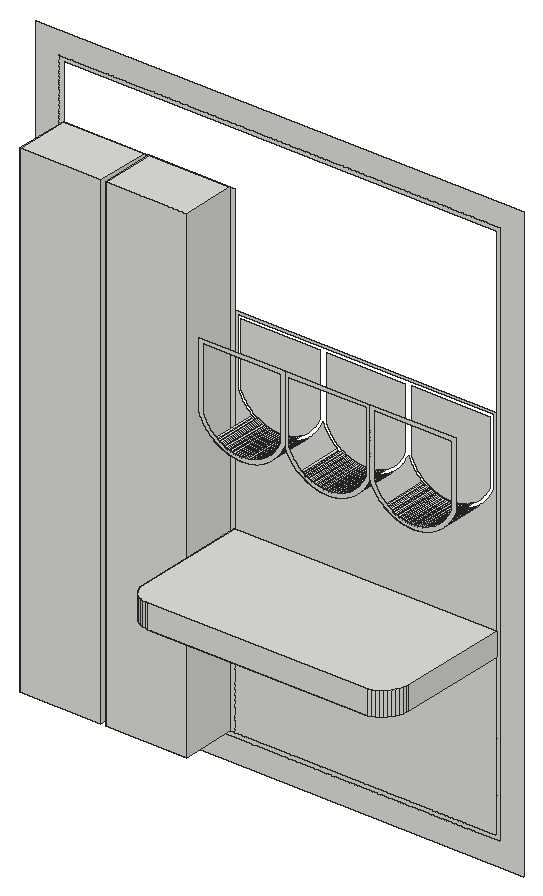
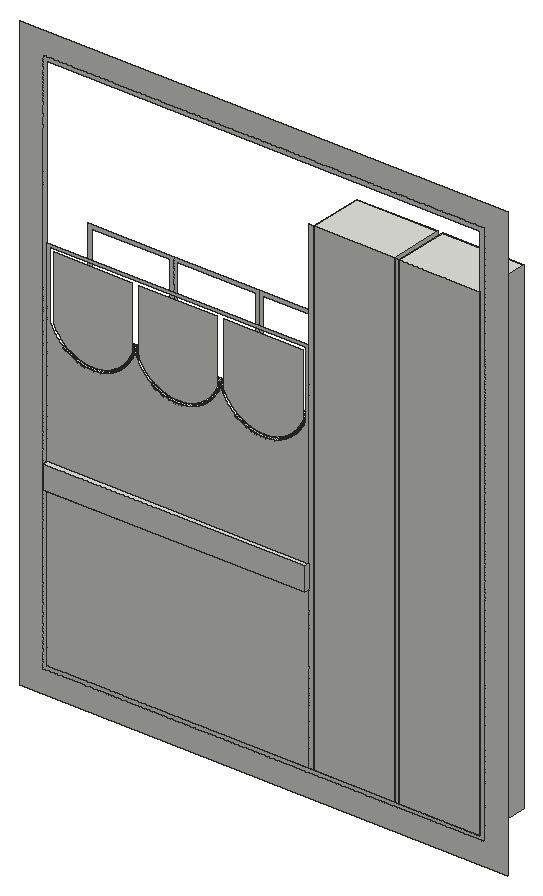
# SketchUp Ruby script. Lengths in inches.
U = 1.inch
M = Sketchup.active_model
def pt(a) = Geom::Point3d.new(a.map { |v| v * U })
def face(e, loops, mat)
  f = e.add_face(loops[0].map { |a| pt(a) })
  loops[1..].each { |l| e.add_face(l.map { |a| pt(a) }).erase! }
  f.material = f.back_material = mat if mat
  f
end
# faces: each face lists its corners as indices into pts; further lists are holes
def faces(e, pts, list, mat = nil) = list.each { |f| face(e, (f[0].is_a?(Array) ? f : [f]).map { |l| l.map { |i| pts[i] } }, mat) }
# xy, xz, yz: faces in a plane at the given z, y or x. An outline is a flat list of corners, or four numbers for a rectangle; further outlines are holes
def ring(l) = l.size == 4 ? [[l[0], l[1]], [l[2], l[1]], [l[2], l[3]], [l[0], l[3]]] : l.each_slice(2).to_a
def flat(e, list, mat, &to3) = list.each { |f| face(e, (f[0].is_a?(Array) ? f : [f]).map { |l| ring(l).map { |u, v| to3.(u, v) } }, mat) }
def xy(e, z, list, mat = nil) = flat(e, list, mat) { |x, y| [x, y, z] }
def xz(e, y, list, mat = nil) = flat(e, list, mat) { |x, z| [x, y, z] }
def yz(e, x, list, mat = nil) = flat(e, list, mat) { |y, z| [x, y, z] }
def lines(e, pts, list) = list.each { |a, b| e.add_line(pt(pts[a]), pt(pts[b])) }
# prism: a flat outline (further loops are holes) pulled along v
def prism(e, loops, v, mat = nil)
  f = face(e, loops, mat); d = Geom::Vector3d.new(v.map { |x| x * U })
  f.pushpull(f.normal.samedirection?(d) ? d.length : -d.length)
end
def box(e, o, s, mat = nil) = prism(e, [[o, [o[0] + s[0], o[1], o[2]], [o[0] + s[0], o[1] + s[1], o[2]], [o[0], o[1] + s[1], o[2]]]], [0, 0, s[2]], mat)
def at(x, y, z, deg = 0) = Geom::Transformation.translation(pt([x, y, z])) * Geom::Transformation.rotation(ORIGIN, Z_AXIS, deg.degrees)
def axes(o, x, y, z) = Geom::Transformation.new([*x, 0, *y, 0, *z, 0, *pt(o).to_a, 1])
def part(name) = M.definitions.add(name)
# library, detail: a bought-in or finely detailed component or shape, given as its bounding box
def library(name, o, s) = part(name).tap { |d| box(d.entities, o, s) }
def detail(e, o, s) = box(e.add_group.entities, o, s)
def put(e, d, t, mat = nil) = e.add_instance(d, t).tap { |i| i.material = mat if mat }
def group(e, t, mat = nil) = e.add_group.tap { |g| g.transformation = t; g.material = mat if mat }.entities
root = M.entities
xy(root,62.04,[[91.5625,19.34,91.81,30],[91.81,19.34,92.06,30],[92.06,19.34,92.3,30]])
xy(root,62.1,[[72.875,19.34,73.125,30]])
xy(root,62.12,[[53.94,19.34,54.19,30]])
xy(root,62.84,[[91.59,19.34,91.82,30],[91.82,19.34,92.05,30],[92.05,19.34,92.28,30]])
xy(root,62.9,[[72.89,19.34,73.11,30]])
xy(root,62.92,[[53.73,19.34,53.95,30],[53.95,19.34,54.18,30],[54.18,19.34,54.41,30]])
xz(root,19.34,[[[91.5625,62.04,92.3,62.04,92.55,62.06,92.8,62.07,93.05,62.1,93.29,62.13,93.54,62.17,93.78,62.21,94.26,62.31,94.5,62.37,94.74,62.4375,94.98,62.51,95.22,62.59,95.45,62.67,95.91,62.85,96.13,62.95,96.36,63.06,96.58,63.17,96.8,63.29,97.01,63.41,97.23,63.53,97.4375,63.67,97.64,63.8,97.84,63.95,98.04,64.09,98.24,64.25,98.43,64.4,98.62,64.5625,98.8,64.73,99.16,65.07,99.33,65.25,99.49,65.4375,99.66,65.625,99.8125,65.81,99.97,66.01,100.11,66.21,100.26,66.41,100.4,66.62,100.53,66.82,100.66,67.04,100.78,67.25,100.9,67.47,101.01,67.69,101.11,67.91,101.15,68,101.21,68.14,101.31,68.37,101.4,68.6,101.4,83.4,82.47,83.4,82.47,68.6,82.65,68.14,82.71,68,82.75,67.91,82.97,67.47,83.09,67.25,83.21,67.04,83.34,66.82,83.47,66.62,83.61,66.41,83.75,66.21,84.05,65.81,84.21,65.625,84.37,65.4375,84.54,65.25,84.71,65.07,84.89,64.9,85.06,64.73,85.25,64.5625,85.4375,64.4,85.63,64.25,85.82,64.09,86.02,63.95,86.22,63.8,86.43,63.67,86.64,63.53,86.85,63.41,87.29,63.17,87.73,62.95,87.96,62.85,88.1875,62.76,88.42,62.67,88.65,62.59,88.89,62.51,89.125,62.4375,89.36,62.37,89.6,62.31,89.84,62.26,90.09,62.21,90.33,62.17,90.58,62.13,90.82,62.1,91.07,62.07,91.31,62.06],[91.59,62.84,91.36,62.86,91.14,62.87,90.91,62.89,90.68,62.92,90.46,62.96,90.23,62.99,89.57,63.14,89.35,63.2,88.91,63.34,88.7,63.42,88.48,63.5,88.27,63.59,88.0625,63.68,87.86,63.78,87.65,63.88,87.25,64.1,86.68,64.46,86.49,64.59,86.31,64.73,86.125,64.87,85.95,65.01,85.78,65.16,85.61,65.32,85.44,65.47,85.28,65.63,84.97,65.97,84.82,66.14,84.4,66.68,84.27,66.86,84.14,67.05,84.02,67.25,83.9,67.44,83.68,67.84,83.58,68.04,83.48,68.25,83.45,68.33,83.39,68.46,83.3,68.67,83.27,68.75,83.27,82.6,100.6,82.6,100.6,68.75,100.57,68.67,100.48,68.46,100.42,68.33,100.39,68.25,100.29,68.04,100.1875,67.84,100.08,67.64,99.97,67.44,99.85,67.25,99.73,67.05,99.6,66.86,99.47,66.68,99.05,66.14,98.9,65.97,98.74,65.8,98.59,65.63,98.42,65.47,98.26,65.32,98.09,65.16,97.92,65.01,97.56,64.73,97.375,64.59,97.19,64.46,96.81,64.22,96.61,64.1,96.21,63.88,96.01,63.78,95.8,63.68,95.38,63.5,94.96,63.34,94.52,63.2,94.3,63.14,93.86,63.04,93.63,62.99,93.41,62.96,93.18,62.92,92.96,62.89,92.73,62.87,92.5,62.86,92.28,62.84]],[[72.875,62.1,73.125,62.1,73.37,62.11,73.62,62.12,73.86,62.14,74.11,62.16,74.35,62.1875,74.6,62.23,75.08,62.31,75.32,62.37,75.5625,62.43,75.8,62.49,76.04,62.5625,76.27,62.64,76.5,62.72,76.73,62.8125,76.96,62.9,77.1875,63,77.41,63.11,77.85,63.33,78.0625,63.45,78.28,63.58,78.49,63.71,79.09,64.13,79.29,64.28,79.48,64.4375,79.67,64.6,79.85,64.76,80.21,65.1,80.55,65.46,80.87,65.84,81.02,66.03,81.17,66.23,81.3125,66.43,81.45,66.63,81.84,67.26,81.96,67.48,82.18,67.92,82.21,68,82.28,68.14,82.47,68.6,82.47,83.4,63.53,83.4,63.53,68.6,63.72,68.14,63.79,68,63.82,67.92,64.04,67.48,64.16,67.26,64.55,66.63,64.6875,66.43,64.83,66.23,64.98,66.03,65.13,65.84,65.45,65.46,65.79,65.1,66.15,64.76,66.33,64.6,66.52,64.4375,66.71,64.28,66.91,64.13,67.51,63.71,67.72,63.58,67.9375,63.45,68.15,63.33,68.59,63.11,68.8125,63,69.04,62.9,69.27,62.8125,69.5,62.72,69.73,62.64,69.96,62.5625,70.2,62.49,70.4375,62.43,70.68,62.37,70.92,62.31,71.4,62.23,71.65,62.1875,71.89,62.16,72.14,62.14,72.38,62.12,72.63,62.11],[72.89,62.9,72.43,62.92,72.21,62.93,71.98,62.95,71.75,62.98,71.53,63.02,71.31,63.05,71.08,63.1,70.64,63.2,70.42,63.26,70.2,63.33,69.99,63.4,69.77,63.47,69.5625,63.55,69.35,63.64,69.14,63.73,68.9375,63.83,68.73,63.93,68.53,64.04,68.34,64.15,68.14,64.26,67.95,64.38,67.57,64.64,67.39,64.77,67.03,65.05,66.86,65.2,66.6875,65.35,66.52,65.51,66.2,65.83,65.75,66.34,65.61,66.52,65.48,66.7,65.34,66.89,65.22,67.07,65.09,67.27,64.97,67.46,64.86,67.66,64.75,67.85,64.65,68.06,64.55,68.26,64.52,68.33,64.45,68.47,64.33,68.75,64.33,82.6,81.67,82.6,81.67,68.75,81.55,68.47,81.48,68.33,81.45,68.26,81.35,68.06,81.25,67.85,81.14,67.66,81.03,67.46,80.91,67.27,80.78,67.07,80.66,66.89,80.52,66.7,80.39,66.52,80.25,66.34,79.8,65.83,79.48,65.51,79.3125,65.35,79.14,65.2,78.97,65.05,78.61,64.77,78.43,64.64,78.05,64.38,77.86,64.26,77.66,64.15,77.47,64.04,77.27,63.93,77.0625,63.83,76.86,63.73,76.65,63.64,76.4375,63.55,76.23,63.47,76.01,63.4,75.8,63.33,75.58,63.26,75.36,63.2,74.92,63.1,74.69,63.05,74.47,63.02,74.25,62.98,74.02,62.95,73.79,62.93,73.57,62.92,73.11,62.9]],[[53.94,62.12,54.19,62.12,54.4375,62.125,54.68,62.14,54.93,62.15,55.17,62.18,55.42,62.21,55.66,62.24,55.9,62.29,56.15,62.33,56.39,62.39,56.86,62.51,57.1,62.58,57.33,62.66,57.57,62.74,57.8,62.83,58.02,62.92,58.25,63.02,58.69,63.23,58.91,63.35,59.34,63.59,59.55,63.72,60.15,64.14,60.35,64.29,60.73,64.61,60.91,64.77,61.27,65.11,61.61,65.47,61.77,65.66,61.93,65.84,62.08,66.04,62.23,66.23,62.375,66.43,62.51,66.64,62.65,66.84,62.78,67.05,62.9,67.27,63.02,67.48,63.28,68,63.34,68.15,63.44,68.37,63.53,68.6,63.53,83.4,44.6,83.4,44.6,68.6,44.69,68.37,44.79,68.15,44.86,68,44.89,67.92,45.11,67.48,45.23,67.27,45.36,67.05,45.49,66.84,45.62,66.64,45.76,66.43,45.9,66.23,46.05,66.04,46.21,65.84,46.36,65.66,46.53,65.47,46.69,65.29,47.04,64.94,47.22,64.77,47.4,64.61,47.78,64.29,47.98,64.14,48.38,63.86,48.59,63.72,48.8,63.59,49.22,63.35,49.44,63.23,49.88,63.02,50.11,62.92,50.57,62.74,51.03,62.58,51.27,62.51,51.99,62.33,52.23,62.29,52.47,62.24,52.72,62.21,52.96,62.18,53.21,62.15,53.45,62.14,53.7,62.125],[53.73,62.92,53.5,62.93,53.27,62.95,53.05,62.97,52.82,63,52.6,63.03,52.375,63.07,52.15,63.12,51.93,63.16,51.27,63.34,51.06,63.41,50.84,63.49,50.63,63.57,50.21,63.75,50.01,63.84,49.81,63.94,49.6,64.05,49.41,64.16,49.21,64.28,48.83,64.52,48.64,64.65,48.46,64.78,48.28,64.92,48.1,65.07,47.93,65.21,47.76,65.36,47.59,65.52,47.27,65.84,46.97,66.18,46.83,66.35,46.68,66.53,46.55,66.71,46.41,66.89,46.29,67.08,46.16,67.27,46.04,67.46,45.71,68.06,45.61,68.26,45.4,68.75,45.4,82.6,62.73,82.6,62.73,68.75,62.52,68.26,62.42,68.06,62.3125,67.86,62.2,67.66,62.09,67.46,61.85,67.08,61.72,66.89,61.59,66.71,61.31,66.35,60.86,65.84,60.54,65.52,60.375,65.36,60.2,65.21,60.03,65.07,59.85,64.92,59.67,64.78,59.49,64.65,59.3,64.52,58.73,64.16,58.33,63.94,58.125,63.84,57.92,63.75,57.5,63.57,57.08,63.41,56.86,63.34,56.2,63.16,55.98,63.12,55.76,63.07,55.54,63.03,55.3125,63,55.09,62.97,54.63,62.93,54.41,62.92]]])
xz(root,30,[[[0,-6,108,126],[5,-1,103,121]],[[5,-1,103,121],[6,0,102,120]],[24,0,25,108],[43,0,44,108],[44,0,102,35.4],
  [[44,40.6,102,84],[91.5625,62.04,91.31,62.06,91.07,62.07,90.82,62.1,90.58,62.13,90.33,62.17,90.09,62.21,89.84,62.26,89.6,62.31,89.36,62.37,89.125,62.4375,88.89,62.51,88.65,62.59,88.42,62.67,88.1875,62.76,87.96,62.85,87.73,62.95,87.29,63.17,86.85,63.41,86.64,63.53,86.43,63.67,86.22,63.8,86.02,63.95,85.82,64.09,85.63,64.25,85.4375,64.4,85.25,64.5625,85.06,64.73,84.89,64.9,84.71,65.07,84.54,65.25,84.37,65.4375,84.21,65.625,84.05,65.81,83.75,66.21,83.61,66.41,83.47,66.62,83.34,66.82,83.21,67.04,83.09,67.25,82.97,67.47,82.75,67.91,82.71,68,82.65,68.14,82.47,68.6,82.28,68.14,82.21,68,82.18,67.92,81.96,67.48,81.84,67.26,81.45,66.63,81.3125,66.43,81.17,66.23,81.02,66.03,80.87,65.84,80.55,65.46,80.21,65.1,79.85,64.76,79.67,64.6,79.48,64.4375,79.29,64.28,79.09,64.13,78.49,63.71,78.28,63.58,78.0625,63.45,77.85,63.33,77.41,63.11,77.1875,63,76.96,62.9,76.73,62.8125,76.5,62.72,76.27,62.64,76.04,62.5625,75.8,62.49,75.5625,62.43,75.32,62.37,75.08,62.31,74.6,62.23,74.35,62.1875,74.11,62.16,73.86,62.14,73.62,62.12,73.37,62.11,73.125,62.1,72.875,62.1,72.63,62.11,72.38,62.12,72.14,62.14,71.89,62.16,71.65,62.1875,71.4,62.23,70.92,62.31,70.68,62.37,70.4375,62.43,70.2,62.49,69.96,62.5625,69.73,62.64,69.5,62.72,69.27,62.8125,69.04,62.9,68.8125,63,68.59,63.11,68.15,63.33,67.9375,63.45,67.72,63.58,67.51,63.71,66.91,64.13,66.71,64.28,66.52,64.4375,66.33,64.6,66.15,64.76,65.79,65.1,65.45,65.46,65.13,65.84,64.98,66.03,64.83,66.23,64.6875,66.43,64.55,66.63,64.16,67.26,64.04,67.48,63.82,67.92,63.79,68,63.72,68.14,63.53,68.6,63.44,68.37,63.34,68.15,63.28,68,63.02,67.48,62.9,67.27,62.78,67.05,62.65,66.84,62.51,66.64,62.375,66.43,62.23,66.23,62.08,66.04,61.93,65.84,61.77,65.66,61.61,65.47,61.27,65.11,60.91,64.77,60.73,64.61,60.35,64.29,60.15,64.14,59.55,63.72,59.34,63.59,58.91,63.35,58.69,63.23,58.25,63.02,58.02,62.92,57.8,62.83,57.57,62.74,57.33,62.66,57.1,62.58,56.86,62.51,56.39,62.39,56.15,62.33,55.9,62.29,55.66,62.24,55.42,62.21,55.17,62.18,54.93,62.15,54.68,62.14,54.4375,62.125,54.19,62.12,53.94,62.12,53.7,62.125,53.45,62.14,53.21,62.15,52.96,62.18,52.72,62.21,52.47,62.24,52.23,62.29,51.99,62.33,51.27,62.51,51.03,62.58,50.57,62.74,50.11,62.92,49.88,63.02,49.44,63.23,49.22,63.35,48.8,63.59,48.59,63.72,48.38,63.86,47.98,64.14,47.78,64.29,47.4,64.61,47.22,64.77,47.04,64.94,46.69,65.29,46.53,65.47,46.36,65.66,46.21,65.84,46.05,66.04,45.9,66.23,45.76,66.43,45.62,66.64,45.49,66.84,45.36,67.05,45.23,67.27,45.11,67.48,44.89,67.92,44.86,68,44.79,68.15,44.69,68.37,44.6,68.6,44.6,83.4,101.4,83.4,101.4,68.6,101.31,68.37,101.21,68.14,101.15,68,101.11,67.91,101.01,67.69,100.9,67.47,100.78,67.25,100.66,67.04,100.53,66.82,100.4,66.62,100.26,66.41,100.11,66.21,99.97,66.01,99.8125,65.81,99.66,65.625,99.49,65.4375,99.33,65.25,99.16,65.07,98.8,64.73,98.62,64.5625,98.43,64.4,98.24,64.25,98.04,64.09,97.84,63.95,97.64,63.8,97.4375,63.67,97.23,63.53,97.01,63.41,96.8,63.29,96.58,63.17,96.36,63.06,96.13,62.95,95.91,62.85,95.45,62.67,95.22,62.59,94.98,62.51,94.74,62.4375,94.5,62.37,94.26,62.31,93.78,62.21,93.54,62.17,93.29,62.13,93.05,62.1,92.8,62.07,92.55,62.06,92.3,62.04]],[91.59,62.84,92.28,62.84,92.5,62.86,92.73,62.87,92.96,62.89,93.18,62.92,93.41,62.96,93.63,62.99,93.86,63.04,94.3,63.14,94.52,63.2,94.96,63.34,95.38,63.5,95.8,63.68,96.01,63.78,96.21,63.88,96.61,64.1,96.81,64.22,97.19,64.46,97.375,64.59,97.56,64.73,97.92,65.01,98.09,65.16,98.26,65.32,98.42,65.47,98.59,65.63,98.74,65.8,98.9,65.97,99.05,66.14,99.47,66.68,99.6,66.86,99.73,67.05,99.85,67.25,99.97,67.44,100.08,67.64,100.1875,67.84,100.29,68.04,100.39,68.25,100.42,68.33,100.48,68.46,100.57,68.67,100.6,68.75,100.6,82.6,83.27,82.6,83.27,68.75,83.3,68.67,83.39,68.46,83.45,68.33,83.48,68.25,83.58,68.04,83.68,67.84,83.9,67.44,84.02,67.25,84.14,67.05,84.27,66.86,84.4,66.68,84.82,66.14,84.97,65.97,85.28,65.63,85.44,65.47,85.61,65.32,85.78,65.16,85.95,65.01,86.125,64.87,86.31,64.73,86.49,64.59,86.68,64.46,87.25,64.1,87.65,63.88,87.86,63.78,88.0625,63.68,88.27,63.59,88.48,63.5,88.7,63.42,88.91,63.34,89.35,63.2,89.57,63.14,90.23,62.99,90.46,62.96,90.68,62.92,90.91,62.89,91.14,62.87,91.36,62.86],[72.89,62.9,73.11,62.9,73.57,62.92,73.79,62.93,74.02,62.95,74.25,62.98,74.47,63.02,74.69,63.05,74.92,63.1,75.36,63.2,75.58,63.26,75.8,63.33,76.01,63.4,76.23,63.47,76.4375,63.55,76.65,63.64,76.86,63.73,77.0625,63.83,77.27,63.93,77.47,64.04,77.66,64.15,77.86,64.26,78.05,64.38,78.43,64.64,78.61,64.77,78.97,65.05,79.14,65.2,79.3125,65.35,79.48,65.51,79.8,65.83,80.25,66.34,80.39,66.52,80.52,66.7,80.66,66.89,80.78,67.07,80.91,67.27,81.03,67.46,81.14,67.66,81.25,67.85,81.35,68.06,81.45,68.26,81.48,68.33,81.55,68.47,81.67,68.75,81.67,82.6,64.33,82.6,64.33,68.75,64.45,68.47,64.52,68.33,64.55,68.26,64.65,68.06,64.75,67.85,64.86,67.66,64.97,67.46,65.09,67.27,65.22,67.07,65.34,66.89,65.48,66.7,65.61,66.52,65.75,66.34,66.2,65.83,66.52,65.51,66.6875,65.35,66.86,65.2,67.03,65.05,67.39,64.77,67.57,64.64,67.95,64.38,68.14,64.26,68.34,64.15,68.53,64.04,68.73,63.93,68.9375,63.83,69.14,63.73,69.35,63.64,69.5625,63.55,69.77,63.47,69.99,63.4,70.2,63.33,70.42,63.26,70.64,63.2,71.08,63.1,71.31,63.05,71.53,63.02,71.75,62.98,71.98,62.95,72.21,62.93,72.43,62.92],[53.73,62.92,54.41,62.92,54.63,62.93,55.09,62.97,55.3125,63,55.54,63.03,55.76,63.07,55.98,63.12,56.2,63.16,56.86,63.34,57.08,63.41,57.5,63.57,57.92,63.75,58.125,63.84,58.33,63.94,58.73,64.16,59.3,64.52,59.49,64.65,59.67,64.78,59.85,64.92,60.03,65.07,60.2,65.21,60.375,65.36,60.54,65.52,60.86,65.84,61.31,66.35,61.59,66.71,61.72,66.89,61.85,67.08,62.09,67.46,62.2,67.66,62.3125,67.86,62.42,68.06,62.52,68.26,62.73,68.75,62.73,82.6,45.4,82.6,45.4,68.75,45.61,68.26,45.71,68.06,46.04,67.46,46.16,67.27,46.29,67.08,46.41,66.89,46.55,66.71,46.68,66.53,46.83,66.35,46.97,66.18,47.27,65.84,47.59,65.52,47.76,65.36,47.93,65.21,48.1,65.07,48.28,64.92,48.46,64.78,48.64,64.65,48.83,64.52,49.21,64.28,49.41,64.16,49.6,64.05,49.81,63.94,50.01,63.84,50.21,63.75,50.63,63.57,50.84,63.49,51.06,63.41,51.27,63.34,51.93,63.16,52.15,63.12,52.375,63.07,52.6,63.03,52.82,63,53.05,62.97,53.27,62.95,53.5,62.93]])
p = [[91.31,30,62.06],[91.5625,30,62.04],[91.5625,19.34,62.04],[91.31,19.34,62.06],[92.3,30,62.04],[92.55,30,62.06],
  [92.55,19.34,62.06],[92.3,19.34,62.04],[53.21,30,62.15],[53.45,30,62.14],[53.45,19.34,62.14],[53.21,19.34,62.15],
  [53.7,30,62.125],[53.7,19.34,62.125],[53.94,30,62.12],[53.94,19.34,62.12],[54.19,30,62.12],[54.4375,30,62.125],
  [54.4375,19.34,62.125],[54.19,19.34,62.12],[54.68,30,62.14],[54.68,19.34,62.14],[54.93,30,62.15],[54.93,19.34,62.15],
  [71.89,30,62.16],[72.14,30,62.14],[72.14,19.34,62.14],[71.89,19.34,62.16],[72.38,30,62.12],[72.38,19.34,62.12],
  [72.63,30,62.11],[72.63,19.34,62.11],[72.875,30,62.1],[72.875,19.34,62.1],[73.125,30,62.1],[73.37,30,62.11],
  [73.37,19.34,62.11],[73.125,19.34,62.1],[73.62,30,62.12],[73.62,19.34,62.12],[73.86,30,62.14],[73.86,19.34,62.14],
  [74.11,30,62.16],[74.11,19.34,62.16],[90.33,30,62.17],[90.58,30,62.13],[90.58,19.34,62.13],[90.33,19.34,62.17],
  [90.82,30,62.1],[90.82,19.34,62.1],[91.07,30,62.07],[91.07,19.34,62.07],[92.8,30,62.07],[92.8,19.34,62.07],
  [93.05,30,62.1],[93.05,19.34,62.1],[93.29,30,62.13],[93.29,19.34,62.13],[93.54,30,62.17],[93.54,19.34,62.17],
  [52.23,30,62.29],[52.47,30,62.24],[52.47,19.34,62.24],[52.23,19.34,62.29],[52.72,30,62.21],[52.72,19.34,62.21],
  [52.96,30,62.18],[52.96,19.34,62.18],[55.17,30,62.18],[55.17,19.34,62.18],[55.42,30,62.21],[55.42,19.34,62.21],
  [55.66,30,62.24],[55.66,19.34,62.24],[55.9,30,62.29],[55.9,19.34,62.29],[71.16,30,62.27],[71.4,30,62.23],
  [71.4,19.34,62.23],[71.16,19.34,62.27],[71.65,30,62.1875],[71.65,19.34,62.1875],[74.35,30,62.1875],[74.35,19.34,62.1875],
  [74.6,30,62.23],[74.6,19.34,62.23],[74.84,30,62.27],[74.84,19.34,62.27],[89.84,30,62.26],[90.09,30,62.21],
  [90.09,19.34,62.21],[89.84,19.34,62.26],[93.78,30,62.21],[93.78,19.34,62.21],[94.02,30,62.26],[94.02,19.34,62.26],
  [51.75,30,62.39],[51.99,30,62.33],[51.99,19.34,62.33],[51.75,19.34,62.39],[56.15,30,62.33],[56.15,19.34,62.33],
  [56.39,30,62.39],[56.39,19.34,62.39],[70.68,30,62.37],[70.92,30,62.31],[70.92,19.34,62.31],[70.68,19.34,62.37],
  [75.08,30,62.31],[75.08,19.34,62.31],[75.32,30,62.37],[75.32,19.34,62.37],[89.36,30,62.37],[89.6,30,62.31],
  [89.6,19.34,62.31],[89.36,19.34,62.37],[94.26,30,62.31],[94.26,19.34,62.31],[94.5,30,62.37],[94.5,19.34,62.37],
  [51.27,30,62.51],[51.51,30,62.45],[51.51,19.34,62.45],[51.27,19.34,62.51],[56.625,30,62.45],[56.625,19.34,62.45],
  [56.86,30,62.51],[56.86,19.34,62.51],[70.2,30,62.49],[70.4375,30,62.43],[70.4375,19.34,62.43],[70.2,19.34,62.49],
  [75.5625,30,62.43],[75.5625,19.34,62.43],[75.8,30,62.49],[75.8,19.34,62.49],[88.89,30,62.51],[89.125,30,62.4375],
  [89.125,19.34,62.4375],[88.89,19.34,62.51],[94.74,30,62.4375],[94.74,19.34,62.4375],[94.98,30,62.51],[94.98,19.34,62.51],
  [51.03,30,62.58],[51.03,19.34,62.58],[57.1,30,62.58],[57.1,19.34,62.58],[69.96,30,62.5625],[69.96,19.34,62.5625],
  [76.04,30,62.5625],[76.04,19.34,62.5625],[88.65,30,62.59],[88.65,19.34,62.59],[95.22,30,62.59],[95.22,19.34,62.59],
  [50.8,30,62.66],[50.8,19.34,62.66],[57.33,30,62.66],[57.33,19.34,62.66],[69.5,30,62.72],[69.73,30,62.64],
  [69.73,19.34,62.64],[69.5,19.34,62.72],[76.27,30,62.64],[76.27,19.34,62.64],[76.5,30,62.72],[76.5,19.34,62.72],
  [88.42,30,62.67],[88.42,19.34,62.67],[95.45,30,62.67],[95.45,19.34,62.67],[50.34,30,62.83],[50.57,30,62.74],
  [50.57,19.34,62.74],[50.34,19.34,62.83],[57.57,30,62.74],[57.57,19.34,62.74],[57.8,30,62.83],[57.8,19.34,62.83],
  [69.27,30,62.8125],[69.27,19.34,62.8125],[76.73,30,62.8125],[76.73,19.34,62.8125],[88.1875,30,62.76],[88.1875,19.34,62.76],
  [95.68,30,62.76],[95.68,19.34,62.76],[50.11,30,62.92],[50.11,19.34,62.92],[58.02,30,62.92],[58.02,19.34,62.92],
  [69.04,30,62.9],[69.04,19.34,62.9],[76.96,30,62.9],[76.96,19.34,62.9],[87.96,30,62.85],[87.96,19.34,62.85],
  [91.59,30,62.84],[91.36,30,62.86],[91.36,19.34,62.86],[91.59,19.34,62.84],[92.5,30,62.86],[92.28,30,62.84],
  [92.28,19.34,62.84],[92.5,19.34,62.86],[95.91,30,62.85],[95.91,19.34,62.85],[49.88,30,63.02],[49.88,19.34,63.02],
  [53.5,30,62.93],[53.27,30,62.95],[53.27,19.34,62.95],[53.5,19.34,62.93],[53.73,30,62.92],[53.73,19.34,62.92],
  [54.63,30,62.93],[54.41,30,62.92],[54.41,19.34,62.92],[54.63,19.34,62.93],[54.86,30,62.95],[54.86,19.34,62.95],
  [58.25,30,63.02],[58.25,19.34,63.02],[68.8125,30,63],[68.8125,19.34,63],[72.21,30,62.93],[71.98,30,62.95],
  [71.98,19.34,62.95],[72.21,19.34,62.93],[72.43,30,62.92],[72.43,19.34,62.92],[72.66,30,62.91],[72.66,19.34,62.91],
  [72.89,30,62.9],[72.89,19.34,62.9],[73.34,30,62.91],[73.11,30,62.9],[73.11,19.34,62.9],[73.34,19.34,62.91],
  [73.57,30,62.92],[73.57,19.34,62.92],[73.79,30,62.93],[73.79,19.34,62.93],[74.02,30,62.95],[74.02,19.34,62.95],
  [77.1875,30,63],[77.1875,19.34,63],[87.73,30,62.95],[87.73,19.34,62.95],[90.68,30,62.92],[90.46,30,62.96],
  [90.46,19.34,62.96],[90.68,19.34,62.92],[90.91,30,62.89],[90.91,19.34,62.89],[91.14,30,62.87],[91.14,19.34,62.87],
  [92.73,30,62.87],[92.73,19.34,62.87],[92.96,30,62.89],[92.96,19.34,62.89],[93.18,30,62.92],[93.18,19.34,62.92],
  [93.41,30,62.96],[93.41,19.34,62.96],[96.13,30,62.95],[96.13,19.34,62.95],[49.66,30,63.125],[49.66,19.34,63.125],
  [52.6,30,63.03],[52.375,30,63.07],[52.375,19.34,63.07],[52.6,19.34,63.03],[52.82,30,63],[52.82,19.34,63],
  [53.05,30,62.97],[53.05,19.34,62.97],[55.09,30,62.97],[55.09,19.34,62.97],[55.3125,30,63],[55.3125,19.34,63],
  [55.54,30,63.03],[55.54,19.34,63.03],[55.76,30,63.07],[55.76,19.34,63.07],[58.47,30,63.125],[58.47,19.34,63.125],
  [68.59,30,63.11],[68.59,19.34,63.11],[71.53,30,63.02],[71.31,30,63.05],[71.31,19.34,63.05],[71.53,19.34,63.02],
  [71.75,30,62.98],[71.75,19.34,62.98],[74.25,30,62.98],[74.25,19.34,62.98],[74.47,30,63.02],[74.47,19.34,63.02],
  [74.69,30,63.05],[74.69,19.34,63.05],[77.41,30,63.11],[77.41,19.34,63.11],[87.51,30,63.06],[87.51,19.34,63.06],
  [90.01,30,63.04],[89.79,30,63.09],[89.79,19.34,63.09],[90.01,19.34,63.04],[90.23,30,62.99],[90.23,19.34,62.99],
  [93.63,30,62.99],[93.63,19.34,62.99],[93.86,30,63.04],[93.86,19.34,63.04],[94.08,30,63.09],[94.08,19.34,63.09],
  [96.36,30,63.06],[96.36,19.34,63.06],[49.44,30,63.23],[49.44,19.34,63.23],[52.15,30,63.12],[51.93,30,63.16],
  [51.93,19.34,63.16],[52.15,19.34,63.12],[55.98,30,63.12],[55.98,19.34,63.12],[56.2,30,63.16],[56.2,19.34,63.16],
  [58.69,30,63.23],[58.69,19.34,63.23],[68.37,30,63.22],[68.37,19.34,63.22],[70.86,30,63.15],[70.64,30,63.2],
  [70.64,19.34,63.2],[70.86,19.34,63.15],[71.08,30,63.1],[71.08,19.34,63.1],[74.92,30,63.1],[74.92,19.34,63.1],
  [75.14,30,63.15],[75.14,19.34,63.15],[75.36,30,63.2],[75.36,19.34,63.2],[77.63,30,63.22],[77.63,19.34,63.22],
  [87.29,30,63.17],[87.29,19.34,63.17],[89.57,30,63.14],[89.35,30,63.2],[89.35,19.34,63.2],[89.57,19.34,63.14],
  [94.3,30,63.14],[94.3,19.34,63.14],[94.52,30,63.2],[94.52,19.34,63.2],[96.58,30,63.17],[96.58,19.34,63.17],
  [49.22,30,63.35],[49.22,19.34,63.35],[51.71,30,63.22],[51.49,30,63.28],[51.49,19.34,63.28],[51.71,19.34,63.22],
  [56.42,30,63.22],[56.42,19.34,63.22],[56.64,30,63.28],[56.64,19.34,63.28],[58.91,30,63.35],[58.91,19.34,63.35],
  [68.15,30,63.33],[68.15,19.34,63.33],[70.42,30,63.26],[70.42,19.34,63.26],[75.58,30,63.26],[75.58,19.34,63.26],
  [77.85,30,63.33],[77.85,19.34,63.33],[87.07,30,63.29],[87.07,19.34,63.29],[89.13,30,63.27],[89.13,19.34,63.27],
  [94.74,30,63.27],[94.74,19.34,63.27],[96.8,30,63.29],[96.8,19.34,63.29],[49.01,30,63.47],[49.01,19.34,63.47],
  [51.27,30,63.34],[51.06,30,63.41],[51.06,19.34,63.41],[51.27,19.34,63.34],[56.86,30,63.34],[56.86,19.34,63.34],
  [57.08,30,63.41],[57.08,19.34,63.41],[59.125,30,63.47],[59.125,19.34,63.47],[67.9375,30,63.45],[67.9375,19.34,63.45],
  [70.2,30,63.33],[69.99,30,63.4],[69.99,19.34,63.4],[70.2,19.34,63.33],[75.8,30,63.33],[75.8,19.34,63.33],
  [76.01,30,63.4],[76.01,19.34,63.4],[78.0625,30,63.45],[78.0625,19.34,63.45],[86.85,30,63.41],[86.85,19.34,63.41],
  [88.91,30,63.34],[88.7,30,63.42],[88.7,19.34,63.42],[88.91,19.34,63.34],[94.96,30,63.34],[94.96,19.34,63.34],
  [95.17,30,63.42],[95.17,19.34,63.42],[97.01,30,63.41],[97.01,19.34,63.41],[50.84,30,63.49],[50.84,19.34,63.49],
  [57.29,30,63.49],[57.29,19.34,63.49],[69.77,30,63.47],[69.77,19.34,63.47],[76.23,30,63.47],[76.23,19.34,63.47],
  [86.64,30,63.53],[86.64,19.34,63.53],[88.48,30,63.5],[88.48,19.34,63.5],[95.38,30,63.5],[95.38,19.34,63.5],
  [97.23,30,63.53],[97.23,19.34,63.53],[48.8,30,63.59],[48.8,19.34,63.59],[50.63,30,63.57],[50.63,19.34,63.57],
  [57.5,30,63.57],[57.5,19.34,63.57],[59.34,30,63.59],[59.34,19.34,63.59],[67.72,30,63.58],[67.72,19.34,63.58],
  [69.5625,30,63.55],[69.5625,19.34,63.55],[76.4375,30,63.55],[76.4375,19.34,63.55],[78.28,30,63.58],[78.28,19.34,63.58],
  [86.43,30,63.67],[86.43,19.34,63.67],[88.27,30,63.59],[88.27,19.34,63.59],[95.59,30,63.59],[95.59,19.34,63.59],
  [97.4375,30,63.67],[97.4375,19.34,63.67],[48.59,30,63.72],[48.59,19.34,63.72],[50.42,30,63.66],[50.42,19.34,63.66],
  [57.71,30,63.66],[57.71,19.34,63.66],[59.55,30,63.72],[59.55,19.34,63.72],[67.51,30,63.71],[67.51,19.34,63.71],
  [69.35,30,63.64],[69.14,30,63.73],[69.14,19.34,63.73],[69.35,19.34,63.64],[76.65,30,63.64],[76.65,19.34,63.64],
  [76.86,30,63.73],[76.86,19.34,63.73],[78.49,30,63.71],[78.49,19.34,63.71],[88.0625,30,63.68],[88.0625,19.34,63.68],
  [95.8,30,63.68],[95.8,19.34,63.68],[48.38,30,63.86],[48.38,19.34,63.86],[50.21,30,63.75],[50.01,30,63.84],
  [50.01,19.34,63.84],[50.21,19.34,63.75],[57.92,30,63.75],[57.92,19.34,63.75],[58.125,30,63.84],[58.125,19.34,63.84],
  [59.75,30,63.86],[59.75,19.34,63.86],[67.31,30,63.85],[67.31,19.34,63.85],[68.9375,30,63.83],[68.9375,19.34,63.83],
  [77.0625,30,63.83],[77.0625,19.34,63.83],[78.69,30,63.85],[78.69,19.34,63.85],[86.22,30,63.8],[86.22,19.34,63.8],
  [87.86,30,63.78],[87.86,19.34,63.78],[96.01,30,63.78],[96.01,19.34,63.78],[97.64,30,63.8],[97.64,19.34,63.8],
  [49.81,30,63.94],[49.81,19.34,63.94],[58.33,30,63.94],[58.33,19.34,63.94],[67.11,30,63.99],[67.11,19.34,63.99],
  [68.73,30,63.93],[68.73,19.34,63.93],[77.27,30,63.93],[77.27,19.34,63.93],[78.89,30,63.99],[78.89,19.34,63.99],
  [86.02,30,63.95],[86.02,19.34,63.95],[87.65,30,63.88],[87.65,19.34,63.88],[96.21,30,63.88],[96.21,19.34,63.88],
  [97.84,30,63.95],[97.84,19.34,63.95],[48.18,30,64],[48.18,19.34,64],[49.6,30,64.05],[49.6,19.34,64.05],
  [58.53,30,64.05],[58.53,19.34,64.05],[59.95,30,64],[59.95,19.34,64],[68.53,30,64.04],[68.53,19.34,64.04],
  [77.47,30,64.04],[77.47,19.34,64.04],[85.82,30,64.09],[85.82,19.34,64.09],[87.45,30,63.99],[87.45,19.34,63.99],
  [96.41,30,63.99],[96.41,19.34,63.99],[98.04,30,64.09],[98.04,19.34,64.09],[47.98,30,64.14],[47.98,19.34,64.14],
  [60.15,30,64.14],[60.15,19.34,64.14],[66.91,30,64.13],[66.91,19.34,64.13],[68.34,30,64.15],[68.34,19.34,64.15],
  [77.66,30,64.15],[77.66,19.34,64.15],[79.09,30,64.13],[79.09,19.34,64.13],[87.25,30,64.1],[87.25,19.34,64.1],
  [96.61,30,64.1],[96.61,19.34,64.1],[47.78,30,64.29],[47.78,19.34,64.29],[49.41,30,64.16],[49.41,19.34,64.16],
  [58.73,30,64.16],[58.73,19.34,64.16],[60.35,30,64.29],[60.35,19.34,64.29],[66.71,30,64.28],[66.71,19.34,64.28],
  [68.14,30,64.26],[68.14,19.34,64.26],[77.86,30,64.26],[77.86,19.34,64.26],[79.29,30,64.28],[79.29,19.34,64.28],
  [85.63,30,64.25],[85.63,19.34,64.25],[87.06,30,64.22],[87.06,19.34,64.22],[96.81,30,64.22],[96.81,19.34,64.22],
  [98.24,30,64.25],[98.24,19.34,64.25],[49.21,30,64.28],[49.21,19.34,64.28],[58.92,30,64.28],[58.92,19.34,64.28],
  [85.4375,30,64.4],[85.4375,19.34,64.4],[86.87,30,64.34],[86.87,19.34,64.34],[97,30,64.34],[97,19.34,64.34],
  [98.43,30,64.4],[98.43,19.34,64.4],[67.95,30,64.38],[67.95,19.34,64.38]]
faces(root,p,[[0,1,2,3],[4,5,6,7],[8,9,10,11],[9,12,13,10],[12,14,15,13],[16,17,18,19],[17,20,21,18],[20,22,23,21],
  [24,25,26,27],[25,28,29,26],[28,30,31,29],[30,32,33,31],[34,35,36,37],[35,38,39,36],[38,40,41,39],[40,42,43,41],
  [44,45,46,47],[45,48,49,46],[48,50,51,49],[50,0,3,51],[5,52,53,6],[52,54,55,53],[54,56,57,55],[56,58,59,57],
  [60,61,62,63],[61,64,65,62],[64,66,67,65],[66,8,11,67],[22,68,69,23],[68,70,71,69],[70,72,73,71],[72,74,75,73],
  [76,77,78,79],[77,80,81,78],[80,24,27,81],[42,82,83,43],[82,84,85,83],[84,86,87,85],[88,89,90,91],[89,44,47,90],
  [58,92,93,59],[92,94,95,93],[96,97,98,99],[97,60,63,98],[74,100,101,75],[100,102,103,101],[104,105,106,107],[105,76,79,106],
  [86,108,109,87],[108,110,111,109],[112,113,114,115],[113,88,91,114],[94,116,117,95],[116,118,119,117],[120,121,122,123],[121,96,99,122],
  [102,124,125,103],[124,126,127,125],[128,129,130,131],[129,104,107,130],[110,132,133,111],[132,134,135,133],[136,137,138,139],[137,112,115,138],
  [118,140,141,119],[140,142,143,141],[144,120,123,145],[126,146,147,127],[148,128,131,149],[134,150,151,135],[152,136,139,153],[142,154,155,143],
  [156,144,145,157],[146,158,159,147],[160,161,162,163],[161,148,149,162],[150,164,165,151],[164,166,167,165],[168,152,153,169],[154,170,171,155],
  [172,173,174,175],[173,156,157,174],[158,176,177,159],[176,178,179,177],[180,160,163,181],[166,182,183,167],[184,168,169,185],[170,186,187,171],
  [188,172,175,189],[178,190,191,179],[192,180,181,193],[182,194,195,183],[196,184,185,197],[198,199,200,201],[202,203,204,205],[186,206,207,187],
  [208,188,189,209],[210,211,212,213],[214,210,213,215],[216,217,218,219],[220,216,219,221],[190,222,223,191],[224,192,193,225],[226,227,228,229],
  [230,226,229,231],[232,230,231,233],[234,232,233,235],[236,237,238,239],[240,236,239,241],[242,240,241,243],[244,242,243,245],[194,246,247,195],
  [248,196,197,249],[250,251,252,253],[254,250,253,255],[256,254,255,257],[199,256,257,200],[258,202,205,259],[260,258,259,261],[262,260,261,263],
  [264,262,263,265],[206,266,267,207],[268,208,209,269],[270,271,272,273],[274,270,273,275],[276,274,275,277],[211,276,277,212],[278,220,221,279],
  [280,278,279,281],[282,280,281,283],[284,282,283,285],[222,286,287,223],[288,224,225,289],[290,291,292,293],[294,290,293,295],[227,294,295,228],
  [296,244,245,297],[298,296,297,299],[300,298,299,301],[246,302,303,247],[304,248,249,305],[306,307,308,309],[310,306,309,311],[251,310,311,252],
  [312,264,265,313],[314,312,313,315],[316,314,315,317],[266,318,319,267],[320,268,269,321],[322,323,324,325],[271,322,325,272],[326,284,285,327],
  [328,326,327,329],[286,330,331,287],[332,288,289,333],[334,335,336,337],[338,334,337,339],[291,338,339,292],[340,300,301,341],[342,340,341,343],
  [344,342,343,345],[302,346,347,303],[348,304,305,349],[350,351,352,353],[307,350,353,308],[354,316,317,355],[356,354,355,357],[318,358,359,319],
  [360,320,321,361],[362,363,364,365],[323,362,365,324],[366,328,329,367],[368,366,367,369],[330,370,371,331],[372,332,333,373],[335,374,375,336],
  [376,344,345,377],[346,378,379,347],[380,348,349,381],[351,382,383,352],[384,356,357,385],[358,386,387,359],[388,360,361,389],[390,391,392,393],
  [363,390,393,364],[394,368,369,395],[396,394,395,397],[370,398,399,371],[400,372,373,401],[402,403,404,405],[374,402,405,375],[406,376,377,407],
  [408,406,407,409],[378,410,411,379],[412,380,381,413],[414,415,416,417],[382,414,417,383],[418,384,385,419],[420,418,419,421],[386,422,423,387],
  [391,424,425,392],[426,396,397,427],[403,428,429,404],[430,408,409,431],[432,412,413,433],[415,434,435,416],[436,420,421,437],[422,438,439,423],
  [440,388,389,441],[424,442,443,425],[444,426,427,445],[398,446,447,399],[448,400,401,449],[428,450,451,429],[452,430,431,453],[410,454,455,411],
  [456,432,433,457],[434,458,459,435],[460,436,437,461],[438,462,463,439],[464,440,441,465],[442,466,467,443],[468,444,445,469],[446,470,471,447],
  [472,448,449,473],[474,475,476,477],[450,474,477,451],[478,452,453,479],[480,478,479,481],[454,482,483,455],[458,484,485,459],[486,460,461,487],
  [488,464,465,489],[490,491,492,493],[466,490,493,467],[494,468,469,495],[496,494,495,497],[470,498,499,471],[500,472,473,501],[475,502,503,476],
  [504,480,481,505],[482,506,507,483],[508,456,457,509],[484,510,511,485],[512,486,487,513],[462,514,515,463],[491,516,517,492],[518,496,497,519],
  [520,500,501,521],[502,522,523,503],[524,504,505,525],[506,526,527,507],[528,508,509,529],[510,530,531,511],[532,512,513,533],[514,534,535,515],
  [536,488,489,537],[516,538,539,517],[540,518,519,541],[498,542,543,499],[522,544,545,523],[546,524,525,547],[548,528,529,549],[530,550,551,531],
  [552,532,533,553],[534,554,555,535],[556,536,537,557],[542,558,559,543],[560,520,521,561],[544,562,563,545],[564,546,547,565],[526,566,567,527],
  [550,568,569,551],[570,552,553,571],[572,556,557,573],[538,574,575,539],[576,540,541,577],[558,578,579,559],[580,560,561,581],[562,582,583,563],
  [584,564,565,585],[566,586,587,567],[588,548,549,589],[568,590,591,569],[592,570,571,593],[554,594,595,555],[574,596,597,575],[598,576,577,599],
  [600,588,589,601],[590,602,603,591],[604,592,593,605],[594,606,607,595],[582,608,609,583]])
g1 = group(root,at(0,30,-6))
xz(g1,0,[[[0,0,108,132],[5,5,103,127]]])
g2 = group(root,at(6,30,0))
box(g2,[0,-12,0],[18,12,108])
g3 = group(root,at(25,30,0))
box(g3,[0,-12,0],[18,12,108])
g4 = group(root,at(44,30,35.4))
xy(g4,0,[[4.82,-30,4.13,-29.95,3.45,-29.8,2.79,-29.56,2.18,-29.22,1.62,-28.8,1.13,-28.31,0.71,-27.75,0.38,-27.13,0.14,-26.48,0,-25.83,0,1.0625,58,1.0625,58,-24.4375,57.96,-24.89,57.82,-25.59,57.6,-26.27,57.3,-26.93,56.92,-27.54,56.48,-28.11,55.98,-28.62,55.42,-29.07,54.81,-29.46,54.16,-29.77,53.48,-30]])
xy(g4,5.2,[[4.82,-30,53.48,-30,54.16,-29.77,54.81,-29.46,55.42,-29.07,55.98,-28.62,56.48,-28.11,56.92,-27.54,57.3,-26.93,57.6,-26.27,57.82,-25.59,57.96,-24.89,58,-24.4375,58,1.0625,0,1.0625,0,-25.83,0.14,-26.48,0.38,-27.13,0.71,-27.75,1.13,-28.31,1.62,-28.8,2.18,-29.22,2.79,-29.56,3.45,-29.8,4.13,-29.95],[58,-24.4375,58.02,-24.17,58,-23.45]])
xz(g4,-30,[[4.82,0,53.48,5.2]])
xz(g4,1.0625,[[0,0,58,5.2]])
yz(g4,0,[[-25.83,0,1.0625,5.2]])
yz(g4,58,[[-24.4375,0,1.0625,5.2]])
p = [[4.13,-29.95,5.2],[3.45,-29.8,5.2],[3.45,-29.8,0],[4.13,-29.95,0],[4.82,-30,5.2],[4.82,-30,0],
  [54.16,-29.77,5.2],[53.48,-30,5.2],[53.48,-30,0],[54.16,-29.77,0],[2.79,-29.56,5.2],[2.79,-29.56,0],
  [54.81,-29.46,5.2],[54.81,-29.46,0],[2.18,-29.22,5.2],[2.18,-29.22,0],[55.42,-29.07,5.2],[55.42,-29.07,0],
  [1.62,-28.8,5.2],[1.62,-28.8,0],[55.98,-28.62,5.2],[55.98,-28.62,0],[1.13,-28.31,5.2],[1.13,-28.31,0],
  [56.48,-28.11,5.2],[56.48,-28.11,0],[0.71,-27.75,5.2],[0.71,-27.75,0],[56.92,-27.54,5.2],[56.92,-27.54,0],
  [0.38,-27.13,5.2],[0.38,-27.13,0],[57.3,-26.93,5.2],[57.3,-26.93,0],[0.14,-26.48,5.2],[0.14,-26.48,0],
  [57.6,-26.27,5.2],[57.6,-26.27,0],[0,-25.83,5.2],[0,-25.83,0],[57.82,-25.59,5.2],[57.82,-25.59,0],
  [57.96,-24.89,5.2],[57.96,-24.89,0],[58,-24.4375,5.2],[58,-24.4375,0]]
faces(g4,p,[[0,1,2,3],[4,0,3,5],[6,7,8,9],[1,10,11,2],[12,6,9,13],[10,14,15,11],[16,12,13,17],[14,18,19,15],
  [20,16,17,21],[18,22,23,19],[24,20,21,25],[22,26,27,23],[28,24,25,29],[26,30,31,27],[32,28,29,33],[30,34,35,31],
  [36,32,33,37],[34,38,39,35],[40,36,37,41],[42,40,41,43],[44,42,43,45]])
